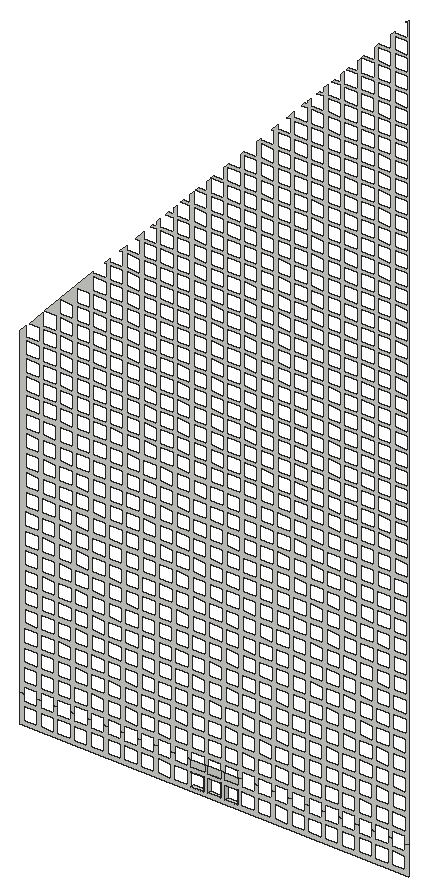
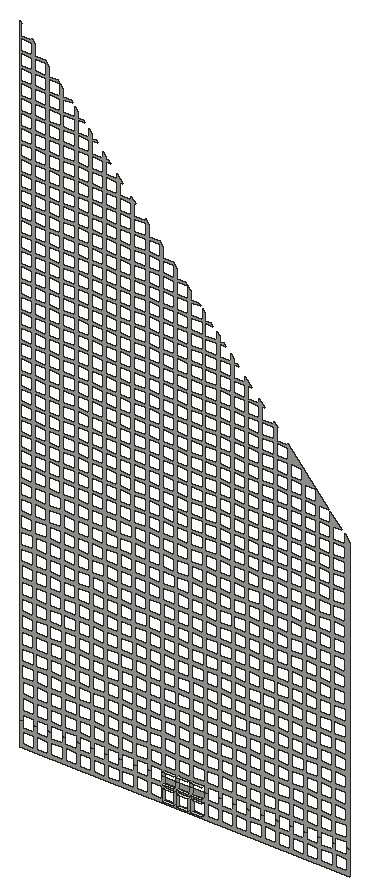
# SketchUp Ruby script. Lengths in inches.
U = 1.inch
M = Sketchup.active_model
def pt(a) = Geom::Point3d.new(a.map { |v| v * U })
def face(e, loops, mat)
  f = e.add_face(loops[0].map { |a| pt(a) })
  loops[1..].each { |l| e.add_face(l.map { |a| pt(a) }).erase! }
  f.material = f.back_material = mat if mat
  f
end
# faces: each face lists its corners as indices into pts; further lists are holes
def faces(e, pts, list, mat = nil) = list.each { |f| face(e, (f[0].is_a?(Array) ? f : [f]).map { |l| l.map { |i| pts[i] } }, mat) }
# xy, xz, yz: faces in a plane at the given z, y or x. An outline is a flat list of corners, or four numbers for a rectangle; further outlines are holes
def ring(l) = l.size == 4 ? [[l[0], l[1]], [l[2], l[1]], [l[2], l[3]], [l[0], l[3]]] : l.each_slice(2).to_a
def flat(e, list, mat, &to3) = list.each { |f| face(e, (f[0].is_a?(Array) ? f : [f]).map { |l| ring(l).map { |u, v| to3.(u, v) } }, mat) }
def xy(e, z, list, mat = nil) = flat(e, list, mat) { |x, y| [x, y, z] }
def xz(e, y, list, mat = nil) = flat(e, list, mat) { |x, z| [x, y, z] }
def yz(e, x, list, mat = nil) = flat(e, list, mat) { |y, z| [x, y, z] }
def lines(e, pts, list) = list.each { |a, b| e.add_line(pt(pts[a]), pt(pts[b])) }
# prism: a flat outline (further loops are holes) pulled along v
def prism(e, loops, v, mat = nil)
  f = face(e, loops, mat); d = Geom::Vector3d.new(v.map { |x| x * U })
  f.pushpull(f.normal.samedirection?(d) ? d.length : -d.length)
end
def box(e, o, s, mat = nil) = prism(e, [[o, [o[0] + s[0], o[1], o[2]], [o[0] + s[0], o[1] + s[1], o[2]], [o[0], o[1] + s[1], o[2]]]], [0, 0, s[2]], mat)
def at(x, y, z, deg = 0) = Geom::Transformation.translation(pt([x, y, z])) * Geom::Transformation.rotation(ORIGIN, Z_AXIS, deg.degrees)
def axes(o, x, y, z) = Geom::Transformation.new([*x, 0, *y, 0, *z, 0, *pt(o).to_a, 1])
def part(name) = M.definitions.add(name)
# library, detail: a bought-in or finely detailed component or shape, given as its bounding box
def library(name, o, s) = part(name).tap { |d| box(d.entities, o, s) }
def detail(e, o, s) = box(e.add_group.entities, o, s)
def put(e, d, t, mat = nil) = e.add_instance(d, t).tap { |i| i.material = mat if mat }
def group(e, t, mat = nil) = e.add_group.tap { |g| g.transformation = t; g.material = mat if mat }.entities
root = M.entities
xy(root,259.68,[[1348.32,480.14,1350.63,480.77],[1351.23,480.14,1353.54,480.77],[1354.14,480.14,1356.45,480.77]])
xy(root,262,[[1348.32,480.14,1350.63,480.77],[1351.23,480.14,1353.54,480.77],[1354.14,480.14,1356.45,480.77]])
xy(root,262.73,[[1348.35,480.14,1350.66,480.77],[1351.26,480.14,1353.57,480.77],[1354.17,480.14,1356.48,480.77]])
xy(root,265.04,[[1348.35,480.14,1350.66,480.77],[1351.26,480.14,1353.57,480.77],[1354.17,480.14,1356.48,480.77]])
xz(root,480.14,[[[1318.58,258.95,1386.17,258.95,1386.17,263.89,1385.6,263.89,1385.6,262.73,1383.29,262.73,1383.29,263.89,1382.69,263.89,1382.69,262.73,1380.38,262.73,1380.38,263.89,1379.78,263.89,1379.78,262.73,1377.47,262.73,1377.47,263.89,1376.87,263.89,1376.87,262.73,1374.56,262.73,1374.56,263.89,1373.96,263.89,1373.96,262.73,1371.64,262.73,1371.64,263.89,1371.04,263.89,1371.04,262.73,1368.73,262.73,1368.73,263.89,1368.13,263.89,1368.13,262.73,1365.82,262.73,1365.82,263.89,1365.22,263.89,1365.22,262.73,1362.91,262.73,1362.91,263.89,1362.31,263.89,1362.31,262.73,1360,262.73,1360,263.89,1359.4,263.89,1359.4,262.73,1357.08,262.73,1357.08,263.89,1356.48,263.89,1356.48,262.73,1354.17,262.73,1354.17,263.89,1353.57,263.89,1353.57,262.73,1351.26,262.73,1351.26,263.89,1350.66,263.89,1350.66,262.73,1348.35,262.73,1348.35,263.89,1347.75,263.89,1347.75,262.73,1345.44,262.73,1345.44,263.89,1344.84,263.89,1344.84,262.73,1342.52,262.73,1342.52,263.89,1341.92,263.89,1341.92,262.73,1339.61,262.73,1339.61,263.89,1339.01,263.89,1339.01,262.73,1336.7,262.73,1336.7,263.89,1336.1,263.89,1336.1,262.73,1333.79,262.73,1333.79,263.89,1333.1875,263.89,1333.1875,262.73,1330.875,262.73,1330.875,263.89,1330.28,263.89,1330.28,262.73,1327.96,262.73,1327.96,263.89,1327.36,263.89,1327.36,262.73,1325.05,262.73,1325.05,263.89,1324.45,263.89,1324.45,262.73,1322.14,262.73,1322.14,263.89,1321.54,263.89,1321.54,262.73,1319.23,262.73,1319.23,263.89,1318.58,263.89],[1383.26,259.68,1385.58,262],[1380.35,259.68,1382.66,262],[1377.4375,259.68,1379.75,262],[1374.53,259.68,1376.84,262],[1371.61,259.68,1373.93,262],[1368.7,259.68,1371.02,262],[1365.79,259.68,1368.1,262],[1362.88,259.68,1365.19,262],[1359.97,259.68,1362.28,262],[1357.05,259.68,1359.37,262],[1354.14,259.68,1356.45,262],[1351.23,259.68,1353.54,262],[1348.32,259.68,1350.63,262],[1345.41,259.68,1347.72,262],[1342.49,259.68,1344.81,262],[1339.58,259.68,1341.89,262],[1336.67,259.68,1338.98,262],[1333.76,259.68,1336.07,262],[1330.85,259.68,1333.16,262],[1327.93,259.68,1330.25,262],[1325.02,259.68,1327.33,262],[1322.11,259.68,1324.42,262],[1319.2,259.68,1321.51,262]],[1348.35,262.73,1350.66,263.89],[1351.26,262.73,1353.57,263.89],[1354.17,262.73,1356.48,263.89],[[1318.58,263.89,1319.23,263.89,1319.23,265.04,1321.54,265.04,1321.54,263.89,1322.14,263.89,1322.14,265.04,1324.45,265.04,1324.45,263.89,1325.05,263.89,1325.05,265.04,1327.36,265.04,1327.36,263.89,1327.96,263.89,1327.96,265.04,1330.28,265.04,1330.28,263.89,1330.875,263.89,1330.875,265.04,1333.1875,265.04,1333.1875,263.89,1333.79,263.89,1333.79,265.04,1336.1,265.04,1336.1,263.89,1336.7,263.89,1336.7,265.04,1339.01,265.04,1339.01,263.89,1339.61,263.89,1339.61,265.04,1341.92,265.04,1341.92,263.89,1342.52,263.89,1342.52,265.04,1344.84,265.04,1344.84,263.89,1345.44,263.89,1345.44,265.04,1347.75,265.04,1347.75,263.89,1348.35,263.89,1348.35,265.04,1350.66,265.04,1350.66,263.89,1351.26,263.89,1351.26,265.04,1353.57,265.04,1353.57,263.89,1354.17,263.89,1354.17,265.04,1356.48,265.04,1356.48,263.89,1357.08,263.89,1357.08,265.04,1359.4,265.04,1359.4,263.89,1360,263.89,1360,265.04,1362.31,265.04,1362.31,263.89,1362.91,263.89,1362.91,265.04,1365.22,265.04,1365.22,263.89,1365.82,263.89,1365.82,265.04,1368.13,265.04,1368.13,263.89,1368.73,263.89,1368.73,265.04,1371.04,265.04,1371.04,263.89,1371.64,263.89,1371.64,265.04,1373.96,265.04,1373.96,263.89,1374.56,263.89,1374.56,265.04,1376.87,265.04,1376.87,263.89,1377.47,263.89,1377.47,265.04,1379.78,265.04,1379.78,263.89,1380.38,263.89,1380.38,265.04,1382.69,265.04,1382.69,263.89,1383.29,263.89,1383.29,265.04,1385.6,265.04,1385.6,263.89,1386.17,263.89,1386.17,392.36,1385.74,391.9,1386.04,391.9,1386.04,389.59,1383.73,389.59,1383.73,389.75,1383.13,389.11,1383.13,386.84,1381,386.84,1380.22,386,1380.22,384.09,1378.42,384.09,1378.1,383.75,1378.01,383.65,1380.22,383.65,1380.22,381.34,1377.9,381.34,1377.9,383.53,1377.3,382.89,1377.3,381.34,1375.84,381.34,1375.43,380.9,1377.3,380.9,1377.3,378.59,1374.99,378.59,1374.99,380.43,1374.39,379.79,1374.39,378.59,1373.27,378.59,1372.86,378.15,1374.39,378.15,1374.39,375.84,1372.08,375.84,1372.08,377.32,1371.48,376.68,1371.48,375.84,1370.6875,375.84,1370.28,375.4,1371.48,375.4,1371.48,373.09,1369.17,373.09,1369.17,374.21,1368.57,373.57,1368.57,373.09,1368.11,373.09,1367.64,372.59,1368.57,372.59,1368.57,370.27,1366.25,370.27,1366.25,371.11,1365.65,370.47,1365.65,370.27,1365.48,370.27,1365.01,369.77,1365.65,369.77,1365.65,367.46,1363.34,367.46,1363.34,368,1362.37,366.96,1362.74,366.96,1362.74,364.65,1360.43,364.65,1360.43,364.89,1359.73,364.15,1359.83,364.15,1359.83,361.84,1357.57,361.84,1356.92,361.14,1356.92,359.02,1354.93,359.02,1354.01,358.04,1354.01,356.21,1352.3,356.21,1351.83,355.71,1354.01,355.71,1354.01,353.4,1351.69,353.4,1351.69,355.57,1351.09,354.93,1351.09,353.4,1349.66,353.4,1349.19,352.9,1351.09,352.9,1351.09,350.59,1348.78,350.59,1348.78,352.46,1348.18,351.82,1348.18,350.59,1347.02,350.59,1346.55,350.09,1348.18,350.09,1348.18,347.77,1345.87,347.77,1345.87,349.36,1345.27,348.72,1345.27,347.77,1344.39,347.77,1343.92,347.27,1345.27,347.27,1345.27,344.96,1342.96,344.96,1342.96,346.25,1342.36,345.61,1342.36,344.96,1341.75,344.96,1341.28,344.46,1342.36,344.46,1342.36,342.15,1340.05,342.15,1340.05,343.14,1338.65,341.65,1339.45,341.65,1339.45,339.34,1337.13,339.34,1337.13,340.04,1336.01,338.84,1336.53,338.84,1336.53,336.52,1334.22,336.52,1334.22,336.93,1333.375,336.02,1333.62,336.02,1333.62,333.71,1331.31,333.71,1331.31,333.82,1322.83,324.77,1324.89,324.77,1324.89,322.46,1322.57,322.46,1322.57,324.5,1320.19,321.96,1321.97,321.96,1321.97,319.65,1319.66,319.65,1319.66,321.39,1318.58,320.24],[1383.73,375.84,1386.04,378.15],[1380.79,373.09,1383.1,375.4],[1383.73,373.09,1386.04,375.4],[1380.79,370.27,1383.1,372.59],[1383.73,370.27,1386.04,372.59],[1372.05,370.27,1374.37,372.59],[1374.99,370.27,1377.3,372.59],[1374.97,373.09,1377.28,375.4],[1377.9,373.09,1380.22,375.4],[1377.88,375.84,1380.19,378.15],[1380.81,375.84,1383.13,378.15],[1380.79,378.59,1383.1,380.9],[1383.73,378.59,1386.04,380.9],[1380.79,381.34,1383.1,383.65],[1383.73,381.34,1386.04,383.65],[1351.69,350.59,1354.01,352.9],[1348.78,347.77,1351.09,350.09],[1351.69,347.77,1354.01,350.09],[1345.87,344.96,1348.18,347.27],[1348.78,344.96,1351.09,347.27],[1351.69,344.96,1354.01,347.27],[1354.61,344.96,1356.92,347.27],[1357.52,344.96,1359.83,347.27],[1360.43,344.96,1362.74,347.27],[1363.34,344.96,1365.65,347.27],[1366.25,344.96,1368.57,347.27],[1369.17,344.96,1371.48,347.27],[1372.08,344.96,1374.39,347.27],[1374.99,344.96,1377.3,347.27],[1377.9,344.96,1380.22,347.27],[1380.81,344.96,1383.13,347.27],[1383.73,344.96,1386.04,347.27],[1354.61,347.77,1356.92,350.09],[1357.52,347.77,1359.83,350.09],[1360.43,347.77,1362.74,350.09],[1363.34,347.77,1365.65,350.09],[1366.25,347.77,1368.57,350.09],[1369.17,347.77,1371.48,350.09],[1372.08,347.77,1374.39,350.09],[1374.99,347.77,1377.3,350.09],[1377.9,347.77,1380.22,350.09],[1380.81,347.77,1383.13,350.09],[1383.73,347.77,1386.04,350.09],[1354.61,350.59,1356.92,352.9],[1357.52,350.59,1359.83,352.9],[1360.43,350.59,1362.74,352.9],[1363.34,350.59,1365.65,352.9],[1366.25,350.59,1368.57,352.9],[1369.17,350.59,1371.48,352.9],[1372.08,350.59,1374.39,352.9],[1374.99,350.59,1377.3,352.9],[1377.9,350.59,1380.22,352.9],[1380.81,350.59,1383.13,352.9],[1383.73,350.59,1386.04,352.9],[1354.61,353.4,1356.92,355.71],[1357.52,353.4,1359.83,355.71],[1360.43,353.4,1362.74,355.71],[1363.34,353.4,1365.65,355.71],[1366.25,353.4,1368.57,355.71],[1369.17,353.4,1371.48,355.71],[1372.08,353.4,1374.39,355.71],[1374.99,353.4,1377.3,355.71],[1377.9,353.4,1380.22,355.71],[1380.81,353.4,1383.13,355.71],[1383.73,353.4,1386.04,355.71],[1366.25,367.46,1368.57,369.77],[1369.17,367.46,1371.48,369.77],[1377.9,367.46,1380.22,369.77],[1383.73,367.46,1386.04,369.77],[1374.99,367.46,1377.3,369.77],[1372.08,367.46,1374.39,369.77],[1380.81,367.46,1383.13,369.77],[1366.25,364.65,1368.57,366.96],[1372.08,364.65,1374.39,366.96],[1380.81,364.65,1383.13,366.96],[1377.9,364.65,1380.22,366.96],[1369.17,364.65,1371.48,366.96],[1374.99,364.65,1377.3,366.96],[1383.73,364.65,1386.04,366.96],[1363.34,364.65,1365.65,366.96],[1374.99,361.84,1377.3,364.15],[1380.81,361.84,1383.13,364.15],[1369.17,361.84,1371.48,364.15],[1372.08,361.84,1374.39,364.15],[1383.73,361.84,1386.04,364.15],[1363.34,361.84,1365.65,364.15],[1360.43,361.84,1362.74,364.15],[1366.25,361.84,1368.57,364.15],[1377.9,361.84,1380.22,364.15],[1374.99,359.02,1377.3,361.34],[1380.81,359.02,1383.13,361.34],[1369.17,359.02,1371.48,361.34],[1357.52,359.02,1359.83,361.34],[1383.73,359.02,1386.04,361.34],[1372.08,359.02,1374.39,361.34],[1363.34,359.02,1365.65,361.34],[1360.43,359.02,1362.74,361.34],[1377.9,359.02,1380.22,361.34],[1366.25,359.02,1368.57,361.34],[1377.9,356.21,1380.22,358.52],[1366.25,356.21,1368.57,358.52],[1360.43,356.21,1362.74,358.52],[1372.08,356.21,1374.39,358.52],[1383.73,356.21,1386.04,358.52],[1354.61,356.21,1356.92,358.52],[1363.34,356.21,1365.65,358.52],[1357.52,356.21,1359.83,358.52],[1369.17,356.21,1371.48,358.52],[1380.81,356.21,1383.13,358.52],[1374.99,356.21,1377.3,358.52],[1342.96,342.15,1345.27,344.46],[1345.87,342.15,1348.18,344.46],[1348.78,342.15,1351.09,344.46],[1351.69,342.15,1354.01,344.46],[1354.61,342.15,1356.92,344.46],[1357.52,342.15,1359.83,344.46],[1360.43,342.15,1362.74,344.46],[1363.34,342.15,1365.65,344.46],[1366.25,342.15,1368.57,344.46],[1369.17,342.15,1371.48,344.46],[1372.08,342.15,1374.39,344.46],[1374.99,342.15,1377.3,344.46],[1377.9,342.15,1380.22,344.46],[1380.81,342.15,1383.13,344.46],[1383.73,342.15,1386.04,344.46],[1340.05,339.34,1342.36,341.65],[1342.96,339.34,1345.27,341.65],[1345.87,339.34,1348.18,341.65],[1348.78,339.34,1351.09,341.65],[1351.69,339.34,1354.01,341.65],[1354.61,339.34,1356.92,341.65],[1357.52,339.34,1359.83,341.65],[1360.43,339.34,1362.74,341.65],[1363.34,339.34,1365.65,341.65],[1366.25,339.34,1368.57,341.65],[1369.17,339.34,1371.48,341.65],[1372.08,339.34,1374.39,341.65],[1374.99,339.34,1377.3,341.65],[1377.9,339.34,1380.22,341.65],[1380.81,339.34,1383.13,341.65],[1383.73,339.34,1386.04,341.65],[1337.13,336.52,1339.45,338.84],[1340.05,336.52,1342.36,338.84],[1342.96,336.52,1345.27,338.84],[1345.87,336.52,1348.18,338.84],[1348.78,336.52,1351.09,338.84],[1351.69,336.52,1354.01,338.84],[1354.61,336.52,1356.92,338.84],[1357.52,336.52,1359.83,338.84],[1360.43,336.52,1362.74,338.84],[1363.34,336.52,1365.65,338.84],[1366.25,336.52,1368.57,338.84],[1369.17,336.52,1371.48,338.84],[1372.08,336.52,1374.39,338.84],[1374.99,336.52,1377.3,338.84],[1377.9,336.52,1380.22,338.84],[1380.81,336.52,1383.13,338.84],[1383.73,336.52,1386.04,338.84],[1334.22,333.71,1336.53,336.02],[1337.13,333.71,1339.45,336.02],[1340.05,333.71,1342.36,336.02],[1342.96,333.71,1345.27,336.02],[1345.87,333.71,1348.18,336.02],[1348.78,333.71,1351.09,336.02],[1351.69,333.71,1354.01,336.02],[1354.61,333.71,1356.92,336.02],[1357.52,333.71,1359.83,336.02],[1360.43,333.71,1362.74,336.02],[1363.34,333.71,1365.65,336.02],[1366.25,333.71,1368.57,336.02],[1369.17,333.71,1371.48,336.02],[1372.08,333.71,1374.39,336.02],[1374.99,333.71,1377.3,336.02],[1377.9,333.71,1380.22,336.02],[1380.81,333.71,1383.13,336.02],[1383.73,333.71,1386.04,336.02],[1331.31,330.9,1333.62,333.21],[1334.22,330.9,1336.53,333.21],[1337.13,330.9,1339.45,333.21],[1340.05,330.9,1342.36,333.21],[1342.96,330.9,1345.27,333.21],[1345.87,330.9,1348.18,333.21],[1348.78,330.9,1351.09,333.21],[1351.69,330.9,1354.01,333.21],[1354.61,330.9,1356.92,333.21],[1357.52,330.9,1359.83,333.21],[1360.43,330.9,1362.74,333.21],[1363.34,330.9,1365.65,333.21],[1366.25,330.9,1368.57,333.21],[1369.17,330.9,1371.48,333.21],[1372.08,330.9,1374.39,333.21],[1374.99,330.9,1377.3,333.21],[1377.9,330.9,1380.22,333.21],[1380.81,330.9,1383.13,333.21],[1383.73,330.9,1386.04,333.21],[1328.4,328.09,1330.71,330.4],[1331.31,328.09,1333.62,330.4],[1334.22,328.09,1336.53,330.4],[1337.13,328.09,1339.45,330.4],[1340.05,328.09,1342.36,330.4],[1342.96,328.09,1345.27,330.4],[1345.87,328.09,1348.18,330.4],[1348.78,328.09,1351.09,330.4],[1351.69,328.09,1354.01,330.4],[1354.61,328.09,1356.92,330.4],[1357.52,328.09,1359.83,330.4],[1360.43,328.09,1362.74,330.4],[1363.34,328.09,1365.65,330.4],[1366.25,328.09,1368.57,330.4],[1369.17,328.09,1371.48,330.4],[1372.08,328.09,1374.39,330.4],[1374.99,328.09,1377.3,330.4],[1377.9,328.09,1380.22,330.4],[1380.81,328.09,1383.13,330.4],[1383.73,328.09,1386.04,330.4],[1325.49,325.27,1327.8,327.59],[1328.4,325.27,1330.71,327.59],[1331.31,325.27,1333.62,327.59],[1334.22,325.27,1336.53,327.59],[1337.13,325.27,1339.45,327.59],[1340.05,325.27,1342.36,327.59],[1342.96,325.27,1345.27,327.59],[1345.87,325.27,1348.18,327.59],[1348.78,325.27,1351.09,327.59],[1351.69,325.27,1354.01,327.59],[1354.61,325.27,1356.92,327.59],[1357.52,325.27,1359.83,327.59],[1360.43,325.27,1362.74,327.59],[1363.34,325.27,1365.65,327.59],[1366.25,325.27,1368.57,327.59],[1369.17,325.27,1371.48,327.59],[1372.08,325.27,1374.39,327.59],[1374.99,325.27,1377.3,327.59],[1377.9,325.27,1380.22,327.59],[1380.81,325.27,1383.13,327.59],[1383.73,325.27,1386.04,327.59],[1325.49,322.46,1327.8,324.77],[1328.4,322.46,1330.71,324.77],[1331.31,322.46,1333.62,324.77],[1334.22,322.46,1336.53,324.77],[1337.13,322.46,1339.45,324.77],[1340.05,322.46,1342.36,324.77],[1342.96,322.46,1345.27,324.77],[1345.87,322.46,1348.18,324.77],[1348.78,322.46,1351.09,324.77],[1351.69,322.46,1354.01,324.77],[1354.61,322.46,1356.92,324.77],[1357.52,322.46,1359.83,324.77],[1360.43,322.46,1362.74,324.77],[1363.34,322.46,1365.65,324.77],[1366.25,322.46,1368.57,324.77],[1369.17,322.46,1371.48,324.77],[1372.08,322.46,1374.39,324.77],[1374.99,322.46,1377.3,324.77],[1377.9,322.46,1380.22,324.77],[1380.81,322.46,1383.13,324.77],[1383.73,322.46,1386.04,324.77],[1322.57,319.65,1324.89,321.96],[1325.49,319.65,1327.8,321.96],[1328.4,319.65,1330.71,321.96],[1331.31,319.65,1333.62,321.96],[1334.22,319.65,1336.53,321.96],[1337.13,319.65,1339.45,321.96],[1340.05,319.65,1342.36,321.96],[1342.96,319.65,1345.27,321.96],[1345.87,319.65,1348.18,321.96],[1348.78,319.65,1351.09,321.96],[1351.69,319.65,1354.01,321.96],[1354.61,319.65,1356.92,321.96],[1357.52,319.65,1359.83,321.96],[1360.43,319.65,1362.74,321.96],[1363.34,319.65,1365.65,321.96],[1366.25,319.65,1368.57,321.96],[1369.17,319.65,1371.48,321.96],[1372.08,319.65,1374.39,321.96],[1374.99,319.65,1377.3,321.96],[1377.9,319.65,1380.22,321.96],[1380.81,319.65,1383.13,321.96],[1383.73,319.65,1386.04,321.96],[1319.66,316.84,1321.97,319.15],[1322.57,316.84,1324.89,319.15],[1325.49,316.84,1327.8,319.15],[1328.4,316.84,1330.71,319.15],[1331.31,316.84,1333.62,319.15],[1334.22,316.84,1336.53,319.15],[1337.13,316.84,1339.45,319.15],[1340.05,316.84,1342.36,319.15],[1342.96,316.84,1345.27,319.15],[1345.87,316.84,1348.18,319.15],[1348.78,316.84,1351.09,319.15],[1351.69,316.84,1354.01,319.15],[1354.61,316.84,1356.92,319.15],[1357.52,316.84,1359.83,319.15],[1360.43,316.84,1362.74,319.15],[1363.34,316.84,1365.65,319.15],[1366.25,316.84,1368.57,319.15],[1369.17,316.84,1371.48,319.15],[1372.08,316.84,1374.39,319.15],[1374.99,316.84,1377.3,319.15],[1377.9,316.84,1380.22,319.15],[1380.81,316.84,1383.13,319.15],[1383.73,316.84,1386.04,319.15],[1319.66,314.02,1321.97,316.34],[1322.57,314.02,1324.89,316.34],[1325.49,314.02,1327.8,316.34],[1328.4,314.02,1330.71,316.34],[1331.31,314.02,1333.62,316.34],[1334.22,314.02,1336.53,316.34],[1337.13,314.02,1339.45,316.34],[1340.05,314.02,1342.36,316.34],[1342.96,314.02,1345.27,316.34],[1345.87,314.02,1348.18,316.34],[1348.78,314.02,1351.09,316.34],[1351.69,314.02,1354.01,316.34],[1354.61,314.02,1356.92,316.34],[1357.52,314.02,1359.83,316.34],[1360.43,314.02,1362.74,316.34],[1363.34,314.02,1365.65,316.34],[1366.25,314.02,1368.57,316.34],[1369.17,314.02,1371.48,316.34],[1372.08,314.02,1374.39,316.34],[1374.99,314.02,1377.3,316.34],[1377.9,314.02,1380.22,316.34],[1380.81,314.02,1383.13,316.34],[1383.73,314.02,1386.04,316.34],[1337.13,311.21,1339.45,313.52],[1340.05,311.21,1342.36,313.52],[1325.49,311.21,1327.8,313.52],[1319.66,311.21,1321.97,313.52],[1380.81,311.21,1383.13,313.52],[1363.34,311.21,1365.65,313.52],[1351.69,311.21,1354.01,313.52],[1328.4,311.21,1330.71,313.52],[1357.52,311.21,1359.83,313.52],[1354.61,311.21,1356.92,313.52],[1331.31,311.21,1333.62,313.52],[1369.17,311.21,1371.48,313.52],[1342.96,311.21,1345.27,313.52],[1377.9,311.21,1380.22,313.52],[1372.08,311.21,1374.39,313.52],[1322.57,311.21,1324.89,313.52],[1366.25,311.21,1368.57,313.52],[1374.99,311.21,1377.3,313.52],[1348.78,311.21,1351.09,313.52],[1383.73,311.21,1386.04,313.52],[1334.22,311.21,1336.53,313.52],[1345.87,311.21,1348.18,313.52],[1360.43,311.21,1362.74,313.52],[1319.66,308.4,1321.97,310.71],[1322.57,308.4,1324.89,310.71],[1325.49,308.4,1327.8,310.71],[1328.4,308.4,1330.71,310.71],[1331.31,308.4,1333.62,310.71],[1334.22,308.4,1336.53,310.71],[1337.13,308.4,1339.45,310.71],[1340.05,308.4,1342.36,310.71],[1342.96,308.4,1345.27,310.71],[1345.87,308.4,1348.18,310.71],[1348.78,308.4,1351.09,310.71],[1351.69,308.4,1354.01,310.71],[1354.61,308.4,1356.92,310.71],[1357.52,308.4,1359.83,310.71],[1360.43,308.4,1362.74,310.71],[1363.34,308.4,1365.65,310.71],[1366.25,308.4,1368.57,310.71],[1369.17,308.4,1371.48,310.71],[1372.08,308.4,1374.39,310.71],[1374.99,308.4,1377.3,310.71],[1377.9,308.4,1380.22,310.71],[1380.81,308.4,1383.13,310.71],[1383.73,308.4,1386.04,310.71],[1319.63,305.35,1321.95,307.67],[1322.54,305.35,1324.86,307.67],[1325.46,305.35,1327.77,307.67],[1328.37,305.35,1330.68,307.67],[1331.28,305.35,1333.59,307.67],[1334.19,305.35,1336.51,307.67],[1337.11,305.35,1339.42,307.67],[1340.02,305.35,1342.33,307.67],[1342.93,305.35,1345.24,307.67],[1345.84,305.35,1348.15,307.67],[1348.75,305.35,1351.07,307.67],[1351.67,305.35,1353.98,307.67],[1354.58,305.35,1356.89,307.67],[1357.49,305.35,1359.8,307.67],[1360.4,305.35,1362.71,307.67],[1363.3125,305.35,1365.625,307.67],[1366.23,305.35,1368.54,307.67],[1369.14,305.35,1371.45,307.67],[1372.05,305.35,1374.36,307.67],[1374.96,305.35,1377.27,307.67],[1377.875,305.35,1380.1875,307.67],[1380.79,305.35,1383.1,307.67],[1383.7,305.35,1386.01,307.67],[1319.6,302.31,1321.92,304.62],[1322.52,302.31,1324.83,304.62],[1325.43,302.31,1327.74,304.62],[1328.34,302.31,1330.65,304.62],[1331.25,302.31,1333.56,304.62],[1334.16,302.31,1336.48,304.62],[1337.08,302.31,1339.39,304.62],[1339.99,302.31,1342.3,304.62],[1342.9,302.31,1345.21,304.62],[1345.8125,302.31,1348.125,304.62],[1348.72,302.31,1351.04,304.62],[1351.64,302.31,1353.95,304.62],[1354.55,302.31,1356.86,304.62],[1357.46,302.31,1359.77,304.62],[1360.37,302.31,1362.68,304.62],[1363.28,302.31,1365.6,304.62],[1366.2,302.31,1368.51,304.62],[1369.11,302.31,1371.42,304.62],[1372.02,302.31,1374.33,304.62],[1374.93,302.31,1377.25,304.62],[1377.84,302.31,1380.16,304.62],[1380.76,302.31,1383.07,304.62],[1383.67,302.31,1385.98,304.62],[1319.57,299.27,1321.89,301.58],[1322.49,299.27,1324.8,301.58],[1325.4,299.27,1327.71,301.58],[1328.3125,299.27,1330.625,301.58],[1331.22,299.27,1333.54,301.58],[1334.14,299.27,1336.45,301.58],[1337.05,299.27,1339.36,301.58],[1339.96,299.27,1342.27,301.58],[1342.87,299.27,1345.18,301.58],[1345.78,299.27,1348.1,301.58],[1348.7,299.27,1351.01,301.58],[1351.61,299.27,1353.92,301.58],[1354.52,299.27,1356.83,301.58],[1357.43,299.27,1359.74,301.58],[1360.34,299.27,1362.66,301.58],[1363.26,299.27,1365.57,301.58],[1366.17,299.27,1368.48,301.58],[1369.08,299.27,1371.39,301.58],[1371.99,299.27,1374.3,301.58],[1374.9,299.27,1377.22,301.58],[1377.82,299.27,1380.13,301.58],[1380.73,299.27,1383.04,301.58],[1383.64,299.27,1385.95,301.58],[1319.55,296.22,1321.86,298.53],[1322.46,296.22,1324.77,298.53],[1325.37,296.22,1327.68,298.53],[1328.28,296.22,1330.59,298.53],[1331.19,296.22,1333.51,298.53],[1334.11,296.22,1336.42,298.53],[1337.02,296.22,1339.33,298.53],[1339.93,296.22,1342.24,298.53],[1342.84,296.22,1345.15,298.53],[1345.75,296.22,1348.07,298.53],[1348.67,296.22,1350.98,298.53],[1351.58,296.22,1353.89,298.53],[1354.49,296.22,1356.8,298.53],[1357.4,296.22,1359.71,298.53],[1360.3125,296.22,1362.625,298.53],[1363.23,296.22,1365.54,298.53],[1366.14,296.22,1368.45,298.53],[1369.05,296.22,1371.36,298.53],[1371.96,296.22,1374.28,298.53],[1374.875,296.22,1377.1875,298.53],[1377.79,296.22,1380.1,298.53],[1380.7,296.22,1383.01,298.53],[1383.61,296.22,1385.92,298.53],[1319.52,293.18,1321.83,295.49],[1322.43,293.18,1324.74,295.49],[1325.34,293.18,1327.65,295.49],[1328.25,293.18,1330.57,295.49],[1331.17,293.18,1333.48,295.49],[1334.08,293.18,1336.39,295.49],[1336.99,293.18,1339.3,295.49],[1339.9,293.18,1342.21,295.49],[1342.8125,293.18,1345.125,295.49],[1345.73,293.18,1348.04,295.49],[1348.64,293.18,1350.95,295.49],[1351.55,293.18,1353.86,295.49],[1354.46,293.18,1356.77,295.49],[1357.375,293.18,1359.6875,295.49],[1360.29,293.18,1362.6,295.49],[1363.2,293.18,1365.51,295.49],[1366.11,293.18,1368.42,295.49],[1369.02,293.18,1371.33,295.49],[1371.93,293.18,1374.25,295.49],[1374.85,293.18,1377.16,295.49],[1377.76,293.18,1380.07,295.49],[1380.67,293.18,1382.98,295.49],[1383.58,293.18,1385.89,295.49],[1319.49,290.13,1321.8,292.44],[1322.4,290.13,1324.71,292.44],[1325.3125,290.13,1327.625,292.44],[1328.22,290.13,1330.54,292.44],[1331.14,290.13,1333.45,292.44],[1334.05,290.13,1336.36,292.44],[1336.96,290.13,1339.27,292.44],[1339.87,290.13,1342.18,292.44],[1342.78,290.13,1345.1,292.44],[1345.7,290.13,1348.01,292.44],[1348.61,290.13,1350.92,292.44],[1351.52,290.13,1353.83,292.44],[1354.43,290.13,1356.74,292.44],[1357.34,290.13,1359.66,292.44],[1360.26,290.13,1362.57,292.44],[1363.17,290.13,1365.48,292.44],[1366.08,290.13,1368.39,292.44],[1368.99,290.13,1371.31,292.44],[1371.9,290.13,1374.22,292.44],[1374.82,290.13,1377.13,292.44],[1377.73,290.13,1380.04,292.44],[1380.64,290.13,1382.95,292.44],[1383.55,290.13,1385.87,292.44],[1319.46,287.09,1321.77,289.4],[1322.37,287.09,1324.68,289.4],[1325.28,287.09,1327.6,289.4],[1328.2,287.09,1330.51,289.4],[1331.11,287.09,1333.42,289.4],[1334.02,287.09,1336.33,289.4],[1336.93,287.09,1339.24,289.4],[1339.84,287.09,1342.16,289.4],[1342.76,287.09,1345.07,289.4],[1345.67,287.09,1347.98,289.4],[1348.58,287.09,1350.89,289.4],[1351.49,287.09,1353.8,289.4],[1354.4,287.09,1356.72,289.4],[1357.32,287.09,1359.63,289.4],[1360.23,287.09,1362.54,289.4],[1363.14,287.09,1365.45,289.4],[1366.05,287.09,1368.36,289.4],[1368.96,287.09,1371.28,289.4],[1371.875,287.09,1374.1875,289.4],[1374.79,287.09,1377.1,289.4],[1377.7,287.09,1380.01,289.4],[1380.61,287.09,1382.92,289.4],[1383.52,287.09,1385.84,289.4],[1319.43,284.04,1321.74,286.35],[1322.34,284.04,1324.65,286.35],[1325.25,284.04,1327.57,286.35],[1328.17,284.04,1330.48,286.35],[1331.08,284.04,1333.39,286.35],[1333.99,284.04,1336.3,286.35],[1336.9,284.04,1339.21,286.35],[1339.8125,284.04,1342.125,286.35],[1342.73,284.04,1345.04,286.35],[1345.64,284.04,1347.95,286.35],[1348.55,284.04,1350.86,286.35],[1351.46,284.04,1353.77,286.35],[1354.375,284.04,1356.6875,286.35],[1357.29,284.04,1359.6,286.35],[1360.2,284.04,1362.51,286.35],[1363.11,284.04,1365.42,286.35],[1366.02,284.04,1368.34,286.35],[1368.93,284.04,1371.25,286.35],[1371.85,284.04,1374.16,286.35],[1374.76,284.04,1377.07,286.35],[1377.67,284.04,1379.98,286.35],[1380.58,284.04,1382.9,286.35],[1383.49,284.04,1385.81,286.35],[1319.4,281,1321.71,283.31],[1322.3125,281,1324.625,283.31],[1325.23,281,1327.54,283.31],[1328.14,281,1330.45,283.31],[1331.05,281,1333.36,283.31],[1333.96,281,1336.27,283.31],[1336.875,281,1339.1875,283.31],[1339.79,281,1342.1,283.31],[1342.7,281,1345.01,283.31],[1345.61,281,1347.92,283.31],[1348.52,281,1350.83,283.31],[1351.43,281,1353.75,283.31],[1354.35,281,1356.66,283.31],[1357.26,281,1359.57,283.31],[1360.17,281,1362.48,283.31],[1363.08,281,1365.39,283.31],[1365.99,281,1368.31,283.31],[1368.91,281,1371.22,283.31],[1371.82,281,1374.13,283.31],[1374.73,281,1377.04,283.31],[1377.64,281,1379.95,283.31],[1380.55,281,1382.87,283.31],[1383.47,281,1385.78,283.31],[1319.37,277.95,1321.68,280.26],[1322.28,277.95,1324.6,280.26],[1325.2,277.95,1327.51,280.26],[1328.11,277.95,1330.42,280.26],[1331.02,277.95,1333.33,280.26],[1333.93,277.95,1336.24,280.26],[1336.84,277.95,1339.16,280.26],[1339.76,277.95,1342.07,280.26],[1342.67,277.95,1344.98,280.26],[1345.58,277.95,1347.89,280.26],[1348.49,277.95,1350.8,280.26],[1351.4,277.95,1353.72,280.26],[1354.32,277.95,1356.63,280.26],[1357.23,277.95,1359.54,280.26],[1360.14,277.95,1362.45,280.26],[1363.05,277.95,1365.36,280.26],[1365.96,277.95,1368.28,280.26],[1368.875,277.95,1371.1875,280.26],[1371.79,277.95,1374.1,280.26],[1374.7,277.95,1377.01,280.26],[1377.61,277.95,1379.93,280.26],[1380.52,277.95,1382.84,280.26],[1383.4375,277.95,1385.75,280.26],[1319.34,274.91,1321.66,277.22],[1322.25,274.91,1324.57,277.22],[1325.17,274.91,1327.48,277.22],[1328.08,274.91,1330.39,277.22],[1330.99,274.91,1333.3,277.22],[1333.9,274.91,1336.22,277.22],[1336.82,274.91,1339.13,277.22],[1339.73,274.91,1342.04,277.22],[1342.64,274.91,1344.95,277.22],[1345.55,274.91,1347.86,277.22],[1348.46,274.91,1350.78,277.22],[1351.375,274.91,1353.6875,277.22],[1354.29,274.91,1356.6,277.22],[1357.2,274.91,1359.51,277.22],[1360.11,274.91,1362.42,277.22],[1363.02,274.91,1365.34,277.22],[1365.9375,274.91,1368.25,277.22],[1368.85,274.91,1371.16,277.22],[1371.76,274.91,1374.07,277.22],[1374.67,274.91,1376.98,277.22],[1377.58,274.91,1379.9,277.22],[1380.5,274.91,1382.81,277.22],[1383.41,274.91,1385.72,277.22],[1319.3125,271.86,1321.625,274.17],[1322.23,271.86,1324.54,274.17],[1325.14,271.86,1327.45,274.17],[1328.05,271.86,1330.36,274.17],[1330.96,271.86,1333.27,274.17],[1333.875,271.86,1336.1875,274.17],[1336.79,271.86,1339.1,274.17],[1339.7,271.86,1342.01,274.17],[1342.61,271.86,1344.92,274.17],[1345.52,271.86,1347.83,274.17],[1348.43,271.86,1350.75,274.17],[1351.35,271.86,1353.66,274.17],[1354.26,271.86,1356.57,274.17],[1357.17,271.86,1359.48,274.17],[1360.08,271.86,1362.39,274.17],[1362.99,271.86,1365.31,274.17],[1365.91,271.86,1368.22,274.17],[1368.82,271.86,1371.13,274.17],[1371.73,271.86,1374.04,274.17],[1374.64,271.86,1376.96,274.17],[1377.55,271.86,1379.87,274.17],[1380.47,271.86,1382.78,274.17],[1383.38,271.86,1385.69,274.17],[1319.28,268.82,1321.6,271.13],[1322.2,268.82,1324.51,271.13],[1325.11,268.82,1327.42,271.13],[1328.02,268.82,1330.33,271.13],[1330.93,268.82,1333.25,271.13],[1333.85,268.82,1336.16,271.13],[1336.76,268.82,1339.07,271.13],[1339.67,268.82,1341.98,271.13],[1342.58,268.82,1344.89,271.13],[1345.49,268.82,1347.81,271.13],[1348.41,268.82,1350.72,271.13],[1351.32,268.82,1353.63,271.13],[1354.23,268.82,1356.54,271.13],[1357.14,268.82,1359.45,271.13],[1360.05,268.82,1362.37,271.13],[1362.97,268.82,1365.28,271.13],[1365.88,268.82,1368.19,271.13],[1368.79,268.82,1371.1,271.13],[1371.7,268.82,1374.01,271.13],[1374.61,268.82,1376.93,271.13],[1377.53,268.82,1379.84,271.13],[1380.4375,268.82,1382.75,271.13],[1383.35,268.82,1385.66,271.13],[1319.26,265.77,1321.57,268.09],[1322.17,265.77,1324.48,268.09],[1325.08,265.77,1327.39,268.09],[1327.99,265.77,1330.3,268.09],[1330.9,265.77,1333.22,268.09],[1333.82,265.77,1336.13,268.09],[1336.73,265.77,1339.04,268.09],[1339.64,265.77,1341.95,268.09],[1342.55,265.77,1344.86,268.09],[1345.46,265.77,1347.78,268.09],[1348.375,265.77,1350.6875,268.09],[1351.29,265.77,1353.6,268.09],[1354.2,265.77,1356.51,268.09],[1357.11,265.77,1359.42,268.09],[1360.02,265.77,1362.34,268.09],[1362.9375,265.77,1365.25,268.09],[1365.85,265.77,1368.16,268.09],[1368.76,265.77,1371.07,268.09],[1371.67,265.77,1373.99,268.09],[1374.58,265.77,1376.9,268.09],[1377.5,265.77,1379.81,268.09],[1380.41,265.77,1382.72,268.09],[1383.32,265.77,1385.63,268.09],[1383.73,384.09,1386.04,386.4],[1380.81,384.09,1383.13,386.4],[1383.73,386.84,1386.04,389.15],[1377.9,370.27,1377.9,372.47,1378.01,372.59,1380.22,372.59,1380.22,370.27],[1369.17,370.27,1369.17,372.47,1369.28,372.59,1371.48,372.59,1371.48,370.27],[1372.08,373.09,1372.08,375.28,1372.1875,375.4,1374.39,375.4,1374.39,373.09],[1374.99,375.84,1374.99,378.03,1375.1,378.15,1377.3,378.15,1377.3,375.84],[1377.9,378.59,1377.9,380.78,1378.01,380.9,1380.22,380.9,1380.22,378.59]]])
yz(root,1350.63,[[480.14,259.68,480.77,262]])
yz(root,1351.23,[[480.14,259.68,480.77,262]])
yz(root,1353.54,[[480.14,259.68,480.77,262]])
yz(root,1354.14,[[480.14,259.68,480.77,262]])
yz(root,1356.45,[[480.14,259.68,480.77,262]])
